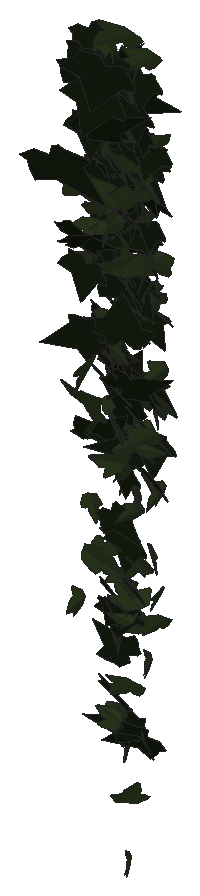
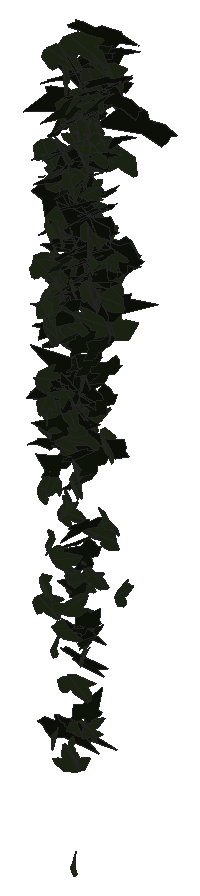
# SketchUp Ruby script. Lengths in millimetres.
U = 1.mm
M = Sketchup.active_model
def pt(a) = Geom::Point3d.new(a.map { |v| v * U })
def face(e, loops, mat)
  f = e.add_face(loops[0].map { |a| pt(a) })
  loops[1..].each { |l| e.add_face(l.map { |a| pt(a) }).erase! }
  f.material = f.back_material = mat if mat
  f
end
# faces: each face lists its corners as indices into pts; further lists are holes
def faces(e, pts, list, mat = nil) = list.each { |f| face(e, (f[0].is_a?(Array) ? f : [f]).map { |l| l.map { |i| pts[i] } }, mat) }
# xy, xz, yz: faces in a plane at the given z, y or x. An outline is a flat list of corners, or four numbers for a rectangle; further outlines are holes
def ring(l) = l.size == 4 ? [[l[0], l[1]], [l[2], l[1]], [l[2], l[3]], [l[0], l[3]]] : l.each_slice(2).to_a
def flat(e, list, mat, &to3) = list.each { |f| face(e, (f[0].is_a?(Array) ? f : [f]).map { |l| ring(l).map { |u, v| to3.(u, v) } }, mat) }
def xy(e, z, list, mat = nil) = flat(e, list, mat) { |x, y| [x, y, z] }
def xz(e, y, list, mat = nil) = flat(e, list, mat) { |x, z| [x, y, z] }
def yz(e, x, list, mat = nil) = flat(e, list, mat) { |y, z| [x, y, z] }
def lines(e, pts, list) = list.each { |a, b| e.add_line(pt(pts[a]), pt(pts[b])) }
# prism: a flat outline (further loops are holes) pulled along v
def prism(e, loops, v, mat = nil)
  f = face(e, loops, mat); d = Geom::Vector3d.new(v.map { |x| x * U })
  f.pushpull(f.normal.samedirection?(d) ? d.length : -d.length)
end
def box(e, o, s, mat = nil) = prism(e, [[o, [o[0] + s[0], o[1], o[2]], [o[0] + s[0], o[1] + s[1], o[2]], [o[0], o[1] + s[1], o[2]]]], [0, 0, s[2]], mat)
def at(x, y, z, deg = 0) = Geom::Transformation.translation(pt([x, y, z])) * Geom::Transformation.rotation(ORIGIN, Z_AXIS, deg.degrees)
def axes(o, x, y, z) = Geom::Transformation.new([*x, 0, *y, 0, *z, 0, *pt(o).to_a, 1])
def part(name) = M.definitions.add(name)
# library, detail: a bought-in or finely detailed component or shape, given as its bounding box
def library(name, o, s) = part(name).tap { |d| box(d.entities, o, s) }
def detail(e, o, s) = box(e.add_group.entities, o, s)
def put(e, d, t, mat = nil) = e.add_instance(d, t).tap { |i| i.material = mat if mat }
def group(e, t, mat = nil) = e.add_group.tap { |g| g.transformation = t; g.material = mat if mat }.entities
root = M.entities
M.materials.add("efeu1").color = [18, 25, 13]
M.materials.add("efeu2").color = [43, 57, 29]
c1 = part("ivyleaf_9")
p = [[39.1,54.8,31.7],[34.5,51.8,30.2],[-5.3,25.2,17.3],[-17.9,28.3,20.9],[-21.6,21.7,17],[-20.2,4.3,5.3],
  [-22.9,-0.3,2.5],[-17.1,-4,-0.6],[-2,-2.1,-1.2],[-0.7,-15.4,-10.1],[16.6,-22.3,-16.7],[21.1,-15.1,-12.5],
  [32.7,-10.7,-11],[46.1,-1.8,-6.6],[30.8,11.2,3.8]]
faces(c1.entities,p,[[0,1,2,3,4,5,6,7,8,9,10,11,12,13,14]],"efeu1")
c2 = part("ivyleaf_10")
p = [[0,12.8,-0.8],[-1.5,51.3,-10.9],[-4.9,51,-11.6],[-13.6,26.5,-7.3],[-13.2,15.9,-4.6],[-21.1,19.3,-7.2],
  [-29.5,16.3,-8.3],[-29.2,8.3,-6.2],[-19.7,-9.8,0.5],[-7.6,-13,4],[1,-12.2,5.8],[-0.4,51.1,-11.1],
  [-1.5,51.1,-10.9],[1,-12.4,5.9],[16.9,-12.4,3.5],[35.1,9.1,-5.1],[35,12.9,-6.1],[20.5,16.4,-4.9],
  [15.8,15,-3.8],[15.3,27.6,-7.1],[12.8,31.3,-7.8]]
faces(c2.entities,p,[[0,1,2,3,4,5,6,7,8,9,10],[11,12,0,13,14,15,16,17,18,19,20]],"efeu2")
put(root,c1,axes([1689.7,958.4,1591.8],[0.18175,-0.69118,-0.44409],[0.28373,0.45424,-0.67492],[1.53762,-0.00212,0.17703]))
put(root,c2,axes([1712.9,944.8,861.4],[0.26339,-0.83853,-0.06256],[-0.02165,0.06153,-0.84988],[1.60018,0.13885,-0.0012]))
put(root,c2,axes([1714.8,968.7,1227.5],[-0.08093,-0.75345,0.21901],[-0.01981,-0.21877,-0.75464],[1.49318,-0.04374,0.00186]))
put(root,c1,axes([1697.6,934.2,1567.8],[0.12261,-0.83473,-0.10782],[-0.03969,0.10651,-0.83712],[1.60137,0.06655,-0.01249]))
put(root,c2,axes([1698,951.7,701.3],[0.88646,-0.26689,0.42385],[0.67692,-0.2313,-0.53649],[0.67121,0.58574,-0.01872]))
put(root,c2,axes([1707.4,908.3,531.4],[-0.11115,-0.03435,0.82545],[0.45417,-0.79293,-0.01611],[1.50533,0.2367,0.06581]))
put(root,c2,axes([1718.6,970.6,1290.3],[-0.64483,-0.74743,0.17146],[-0.05891,-0.17397,-0.81952],[1.45826,-0.33753,0.04271]))
put(root,c2,axes([1712.3,947.3,1230.7],[1.40107,0.27254,-0.1564],[-0.2771,-0.0572,-0.78499],[-0.52997,0.75042,-0.00303]))
put(root,c2,axes([1681.9,953.9,1146.6],[0.09509,-0.01483,0.82486],[1.55484,0.11589,-0.0474],[-0.21851,0.8182,0.02167]))
put(root,c1,axes([1683.9,924.1,1209.7],[0.19618,-0.20205,0.79884],[1.13632,-0.53653,-0.21274],[1.0808,0.60076,0.07867]))
put(root,c2,axes([1694.1,979.8,590.5],[0.81213,-0.23414,-0.46095],[0.7643,-0.22632,0.48672],[-0.61972,-0.58596,-0.0038]))
put(root,c2,axes([1720.6,981.4,1172.7],[-0.21338,-0.76033,0.12533],[-0.03901,-0.12367,-0.76855],[1.46607,-0.11395,-0.00221]))
put(root,c1,axes([1730.8,969.3,1173.4],[-1.32931,-0.39113,0.2691],[0.46256,0.11663,0.80036],[-0.77619,0.73936,0.0161]))
put(root,c1,axes([1692.7,909.5,1210.1],[0.96541,0.73315,-0.17413],[0.18159,0.14573,0.89151],[1.4226,-0.51613,0.00437]))
put(root,c1,axes([1694.9,924,1540.4],[-0.51678,-0.22066,-0.81665],[1.50326,0.24095,-0.32773],[0.57643,-0.82619,0.12253]))
put(root,c1,axes([1697.5,958.3,998.7],[0.37662,-0.72797,0.42536],[0.33819,-0.3911,-0.752],[1.56862,0.2591,0.06]))
put(root,c2,axes([1716.9,959.8,1362.8],[0.0056,0.02601,-0.84155],[0.42991,0.81068,0.02585],[1.54365,-0.22587,-0.00415]))
put(root,c1,axes([1694.8,968.2,942.3],[0.78274,-0.63319,0.40762],[0.43873,-0.33629,-0.75498],[1.3644,0.47139,0.00892]))
put(root,c2,axes([1725.9,907.7,1570.8],[0.01398,-0.83915,0.07771],[0.00221,-0.07771,-0.83918],[1.6039,0.00742,0.00048]))
put(root,c1,axes([1706.2,972.5,1047.1],[0.19524,-0.63407,0.45046],[0.11585,-0.44642,-0.64225],[1.47575,0.11893,-0.00918]))
put(root,c1,axes([1709.6,989,479.4],[0.66706,-0.35539,-0.59071],[0.74817,-0.44134,0.49877],[-1.07779,-0.52632,-0.01937]))
put(root,c2,axes([1725,969.4,1276.2],[0.09274,-0.68093,-0.48319],[0.05434,0.48508,-0.68073],[1.58814,0.02316,0.05151]))
put(root,c2,axes([1725.1,975.1,1174.3],[0.89988,-0.63868,-0.11348],[-0.09706,0.10339,-0.79439],[1.23074,0.47513,0.02032]))
put(root,c1,axes([1716.6,914.3,1171.3],[-0.44413,-0.81643,0.19969],[-0.07124,-0.19695,-0.84894],[1.59805,-0.23568,0.01765]))
put(root,c1,axes([1721.5,989.8,319.3],[0.82818,-0.67144,-0.05441],[0.06196,-0.04374,0.80011],[-1.28057,-0.43636,0.00352]))
put(root,c1,axes([1716.6,976.2,1198.5],[-0.32791,-0.69422,0.4045],[-0.00427,-0.41328,-0.71024],[1.52916,-0.15002,0.08476]))
put(root,c1,axes([1714.3,982.9,1320.9],[-0.00979,-0.79459,-0.01398],[-0.00021,0.01399,-0.79461],[1.5125,-0.00514,-0.0002]))
put(root,c1,axes([1703,980.8,825.3],[0.57062,-0.68673,0.3923],[0.36422,-0.34408,-0.74858],[1.46048,0.35412,0.03341]))
put(root,c1,axes([1721,921.5,1440.8],[-0.45029,-0.78834,0.02024],[-0.00973,-0.0196,-0.82308],[1.50083,-0.23665,0.00074]))
put(root,c2,axes([1723.1,950.8,1264.9],[-0.90653,-0.68564,0.09174],[0.13397,0.06276,0.83457],[-1.30971,0.48099,0.02187]))
put(root,c1,axes([1718.5,995.4,1203.8],[-0.17542,-0.66346,0.40385],[-0.03397,-0.40476,-0.66905],[1.47784,-0.08806,0.03256]))
put(root,c1,axes([1726.3,961.8,1426.7],[-0.70275,-0.70041,0.04303],[-0.02428,-0.04191,-0.79174],[1.33532,-0.36938,0.00825]))
put(root,c1,axes([1714.1,958,1322.9],[0.20442,-0.71739,-0.34234],[0.01173,0.34619,-0.72352],[1.51277,0.09426,0.05187]))
put(root,c1,axes([1714.5,979.5,1246.9],[-0.05502,-0.70997,-0.30148],[0.22795,0.2939,-0.70361],[1.45019,-0.07313,0.09916]))
put(root,c1,axes([1711.7,994.8,505.4],[0.0111,-0.47755,0.6402],[0.33689,-0.62352,-0.46672],[1.48227,0.14529,0.10128]))
put(root,c1,axes([1756.8,971.7,418],[-1.3002,0.00659,-0.40656],[-0.77375,0.0026,0.6832],[0.0133,0.79498,0.00113]))
put(root,c2,axes([1734.7,969.3,1202.3],[0.53911,-0.66026,-0.3094],[-0.12299,0.30789,-0.7162],[1.38227,0.28491,0.05695]))
put(root,c1,axes([1719.2,968.4,1183.5],[1.46545,0.1758,0.2885],[-0.53773,-0.05857,0.78979],[0.35252,-0.82017,0.00544]))
put(root,c1,axes([1703.3,963.2,1259.9],[1.4237,-0.12324,0.3191],[0.59676,-0.05966,-0.7581],[0.26023,0.81108,-0.00728]))
put(root,c1,axes([1716.2,943,829.9],[-0.70545,-0.1078,0.73364],[1.40662,-0.12015,0.35576],[0.11433,0.81313,0.14983]))
put(root,c1,axes([1719.5,949.1,1340],[-0.06274,-0.76151,0.28992],[0.10539,-0.29158,-0.75957],[1.5472,-0.01102,0.0635]))
put(root,c1,axes([1715.1,982.5,1019],[0.28871,-0.66109,0.46611],[0.15423,-0.45943,-0.67798],[1.53173,0.17087,-0.01959]))
put(root,c2,axes([1742.7,975.7,277.2],[0.56167,0.54373,0.45632],[-0.41077,-0.40205,0.61866],[1.28701,-0.36562,-0.00169]))
put(root,c2,axes([1722.2,986.1,294.7],[0.97846,-0.29877,0.32403],[0.53817,-0.15829,-0.5946],[0.64344,0.58673,0.00459]))
put(root,c1,axes([1721.8,958.5,1509.5],[0.02552,-0.80973,0.16957],[0.01297,-0.16948,-0.80983],[1.57445,0.01452,0.00392]))
put(root,c1,axes([1725.2,968.3,1283.7],[-0.91337,0.32252,0.60719],[0.78652,-0.45647,0.56909],[1.04576,0.62501,0.10231]))
put(root,c1,axes([1717.4,970.4,1280.6],[-0.56151,-0.10121,0.8328],[1.58885,0.05168,0.30204],[-0.15752,0.882,0.07787]))
put(root,c2,axes([1728.5,987.5,431.1],[-0.39373,0.19724,0.66334],[0.60116,-0.58911,0.27368],[1.1719,0.36846,0.08247]))
put(root,c2,axes([1728.5,958.7,1446],[0.25264,0.27585,-0.84181],[0.57161,0.78678,0.30518],[1.5861,-0.32748,0.02411]))
put(root,c2,axes([1754.6,968.9,568.4],[-0.60968,-0.19606,-0.6035],[-0.97342,-0.32036,0.37557],[-0.71481,0.60349,0.0033]))
put(root,c1,axes([1769.6,972.8,276.3],[-0.91405,0.24968,0.55378],[-0.93529,0.25528,-0.5413],[-0.67961,-0.68714,0.00012]))
put(root,c2,axes([1741.4,976.4,1441.1],[0.40827,-0.78435,0.05426],[0.0332,-0.05148,-0.81315],[1.49598,0.2152,0.00324]))
put(root,c1,axes([1733.9,996.6,1221.4],[-0.46341,-0.77579,0.29791],[-0.07884,-0.29871,-0.81175],[1.57964,-0.2425,0.04688]))
put(root,c1,axes([1740.8,988.5,490.6],[-1.25205,-0.20013,-0.33798],[0.61416,0.10049,-0.68763],[0.42619,-0.73275,-0.002]))
put(root,c2,axes([1743.6,964.1,1490.1],[0.45172,-0.77855,-0.13077],[-0.05376,0.12809,-0.81386],[1.50153,0.2388,0.0102]))
put(root,c1,axes([1737.9,994.4,1338.5],[-0.62766,-0.68595,0.20589],[-0.07877,-0.20803,-0.7594],[1.36076,-0.32844,0.05101]))
put(root,c1,axes([1727.9,974.1,1162.2],[-0.2298,-0.75737,-0.28282],[0.19594,0.26923,-0.76491],[1.52612,-0.14861,0.05562]))
put(root,c2,axes([1744.7,939.4,1303.3],[0.00013,-0.7838,0.19781],[0.03443,-0.19776,-0.78361],[1.53812,0.00449,0.01752]))
put(root,c2,axes([1746.2,960.2,996.6],[0.46696,-0.40291,-0.73346],[-0.09245,0.75618,-0.43165],[1.58998,0.1623,0.19031]))
put(root,c2,axes([1732.1,937.6,1470.7],[0.68586,-0.63469,0.58028],[0.65757,-0.4693,-0.72788],[1.4988,0.49634,0.0538]))
put(root,c2,axes([1745.3,955.2,980.4],[0.39551,-0.69335,0.09716],[0.06013,-0.09196,-0.72381],[1.33111,0.21017,0.00383]))
put(root,c2,axes([1722,985.9,880.1],[1.06849,-0.05936,0.54914],[1.04372,-0.0334,-0.56427],[0.12526,0.78462,0.01753]))
put(root,c1,axes([1724.3,952.9,1526.3],[0.79877,-0.79627,0.01693],[0.0145,-0.01512,-0.9001],[1.51573,0.41977,-0.00031]))
put(root,c1,axes([1755.9,987.7,944.3],[-1.19985,0.38707,-0.37531],[0.60775,-0.19719,-0.73978],[-0.82676,-0.7067,0.00086]))
put(root,c1,axes([1738.6,944.7,1310.7],[-0.15614,0.39346,0.74912],[-0.18365,-0.75207,0.38445],[1.59991,-0.04793,0.11724]))
put(root,c1,axes([1757.8,874.5,1074.2],[-0.07594,-0.47857,-0.87325],[0.19127,-0.87143,0.47297],[-1.88551,-0.06912,0.08315]))
put(root,c1,axes([1759.8,973.4,820.1],[-0.11583,-0.62189,-0.43502],[-0.09973,-0.43193,0.62481],[-1.44097,0.07989,-0.00827]))
put(root,c2,axes([1736.4,955.2,1301.4],[-0.2989,0.26463,0.78438],[0.77093,-0.6717,0.30772],[1.374,0.43445,-0.00202]))
put(root,c2,axes([1757.2,974.1,1286.5],[-0.60406,-0.62272,0.34803],[-0.21433,-0.33241,-0.69747],[1.34067,-0.33372,0.04531]))
put(root,c1,axes([1724,985.9,1065.8],[0.83335,-0.63856,0.29211],[0.30085,-0.24577,-0.77422],[1.30212,0.46546,-0.00807]))
put(root,c2,axes([1721.9,963.2,1436.4],[1.15835,-0.03301,0.65341],[1.24352,-0.01495,-0.60937],[0.06365,0.89283,0.01395]))
put(root,c1,axes([1746.9,970.3,1545.8],[-0.63528,-0.74643,0.16803],[-0.00823,-0.18148,-0.81477],[1.45612,-0.32668,0.0687]))
put(root,c2,axes([1743.4,951.7,1537.2],[-0.70265,-0.4983,-0.65806],[0.67983,0.55344,-0.61948],[1.41626,-0.51288,-0.02912]))
put(root,c1,axes([1738.5,957.3,687.7],[0.32761,-0.5842,-0.53926],[-0.15922,0.53539,-0.60671],[1.50473,0.18384,0.05321]))
put(root,c1,axes([1735.1,941.7,1527.1],[0.31322,-0.75663,-0.3218],[0.05471,0.33328,-0.76891],[1.56389,0.13988,0.09135]))
put(root,c2,axes([1768.2,967.2,364.2],[-0.95032,-0.27935,0.38802],[-0.63465,-0.1986,-0.57209],[0.6521,-0.60037,0.0087]))
put(root,c2,axes([1756.5,963.3,1482.4],[0.88185,-0.51135,-0.45805],[-0.17449,0.50157,-0.65269],[1.29485,0.41584,0.224]))
put(root,c1,axes([1727.7,968.1,626.1],[0.80692,-0.59008,0.34279],[0.35305,-0.28871,-0.72643],[1.24988,0.46251,-0.01611]))
put(root,c2,axes([1745,994.8,243],[0.59429,-0.53217,0.51218],[0.49076,-0.44253,-0.61701],[1.31725,0.40496,-0.0012]))
put(root,c2,axes([1757.1,926,1558.8],[-0.47647,-0.89449,-0.17919],[0.08701,0.17328,-0.92886],[1.73404,-0.25448,-0.00263]))
put(root,c1,axes([1776.6,961.1,884.9],[-0.04519,0.05329,0.85173],[-0.77536,0.74799,-0.05816],[-1.42715,-0.40807,0.00462]))
put(root,c2,axes([1757.9,968.2,1205.8],[-0.26066,0.64036,0.37512],[-0.39872,0.33258,-0.64423],[-1.355,-0.22105,0.11741]))
put(root,c1,axes([1722.6,968,966.7],[1.30364,-0.22833,0.42596],[0.78395,-0.11064,-0.7217],[0.48111,0.79899,0.02179]))
put(root,c1,axes([1747,980.5,1501],[-0.22377,-0.802,0.12552],[-0.04862,-0.12311,-0.81054],[1.54418,-0.12009,-0.00733]))
put(root,c1,axes([1734.4,973.8,571.3],[0.65266,-0.66391,0.2397],[0.24123,-0.20423,-0.74702],[1.32154,0.36516,0.01799]))
put(root,c2,axes([1763.9,983.8,513.7],[0.72844,0.68648,0.29535],[-0.30241,-0.24949,0.7858],[1.38977,-0.4141,0.01618]))
put(root,c2,axes([1773.1,984.8,469.9],[0.40202,0.25243,0.6061],[-0.75972,-0.45613,0.32909],[0.99211,-0.45158,0.0064]))
put(root,c2,axes([1754.6,938.9,1255.9],[0.15552,-0.302,-0.79484],[0.33589,0.78714,-0.28093],[1.58301,-0.13735,0.1377]))
put(root,c1,axes([1734.8,914.6,1067.5],[0.16697,-0.14272,-0.8229],[1.49898,-0.26113,0.12926],[-0.5288,-0.78528,0.10657]))
put(root,c2,axes([1781.8,938.2,1624.7],[-0.93444,-0.35359,0.63048],[-1.00895,-0.34199,-0.60464],[0.93524,-0.72222,-0.02236]))
put(root,c1,axes([1754.8,969.6,940],[-1.03618,0.47702,0.31955],[0.46198,-0.20784,0.72385],[0.99028,0.59609,-0.00333]))
put(root,c2,axes([1747.4,988.9,10.5],[0.05223,-0.07451,0.68136],[0.69502,-0.57547,-0.07764],[1.10392,0.36584,0.01665]))
put(root,c2,axes([1762.8,977.7,1380.4],[-0.27451,-0.79271,-0.04404],[0.01899,0.04295,-0.80573],[1.5109,-0.14456,0.00213]))
put(root,c1,axes([1772.7,934.8,1348.9],[0.88871,0.12425,-0.72216],[-1.35761,-0.11885,-0.4817],[-0.31909,0.85172,0.03813]))
put(root,c2,axes([1776.8,976.5,917.6],[-1.15502,0.13325,0.44916],[-0.83127,0.10498,-0.6213],[-0.32256,-0.74768,-0.00718]))
put(root,c1,axes([1744.6,963.5,1006.2],[0.15391,-0.70528,0.31233],[0.14915,-0.3049,-0.7088],[1.46042,0.10547,0.03947]))
put(root,c2,axes([1763.9,979.3,1303.3],[-1.34956,-0.36715,-0.06502],[0.10981,0.02998,-0.79851],[0.70108,-0.71145,-0.00009]))
put(root,c1,axes([1750.2,971.7,768],[-0.17442,-0.66778,0.37274],[0.08356,-0.37939,-0.66888],[1.4531,-0.05834,0.0832]))
put(root,c1,axes([1728.5,807.1,1429.7],[-0.28314,-0.30864,-1.04293],[1.57429,0.65139,-0.31076],[1.34408,-0.82797,0.14429]))
put(root,c2,axes([1750.6,981.5,945.8],[1.10286,0.51038,0.1776],[0.24058,0.12515,-0.77213],[-0.99995,0.59302,0.0101]))
put(root,c2,axes([1759.2,971.9,766],[0.3613,-0.66091,0.34813],[0.27021,-0.32073,-0.68631],[1.39577,0.23317,0.04275]))
put(root,c2,axes([1772.4,934.1,1469.3],[-1.58699,0.14332,0.18917],[-0.35391,0.03485,-0.84607],[-0.28066,-0.85433,-0.00278]))
put(root,c2,axes([1746.6,930.1,1601.3],[1.03095,-0.4128,0.53936],[0.8131,-0.32923,-0.68106],[1.00491,0.68989,-0.00228]))
put(root,c2,axes([1751.8,971.3,547.7],[-0.91798,0.13534,0.4645],[0.82941,-0.16334,0.50012],[0.39992,0.64941,0.02899]))
put(root,c2,axes([1754.8,937.9,1429.4],[-1.3764,-0.33241,0.3256],[0.58506,0.11041,0.79552],[-0.66479,0.7854,0.02598]))
put(root,c1,axes([1760.5,951.8,1364.9],[-0.55817,-0.68596,0.31961],[-0.00659,-0.34156,-0.73623],[1.44026,-0.2674,0.1205]))
put(root,c1,axes([1752.6,979.7,1493.2],[0.05627,-0.82043,0.0385],[-0.00986,-0.03871,-0.82094],[1.56313,0.02929,-0.00656]))
put(root,c1,axes([1742.2,985.5,963.7],[0.43339,-0.13195,-0.80412],[1.39862,-0.32752,0.26185],[-0.67013,-0.76889,0.02646]))
put(root,c2,axes([1771.9,944.2,1212.1],[0.80261,-0.55874,-0.39346],[-0.24454,0.38927,-0.69051],[1.2774,0.42558,0.11503]))
put(root,c1,axes([1746.3,953.4,1322],[1.49653,-0.27011,-0.05779],[-0.09921,0.02613,-0.83139],[0.51627,0.78801,0.00775]))
put(root,c1,axes([1737.2,931.2,1035.1],[0.42058,-0.49408,0.66016],[0.86878,-0.49587,-0.52393],[1.30693,0.48863,0.13583]))
put(root,c1,axes([1747.7,953.2,1415.4],[-0.35849,-0.53119,-0.68217],[0.78234,0.5592,-0.54893],[1.44761,-0.43375,0.12773]))
put(root,c1,axes([1755.5,986.3,1361.2],[0.1208,-0.75436,0.21104],[-0.00041,-0.21174,-0.75682],[1.49081,0.06106,-0.01731]))
put(root,c2,axes([1737.5,900.4,630.6],[0.28789,-0.04534,0.82537],[1.57078,-0.03832,-0.15336],[0.08738,0.83824,0.03764]))
put(root,c2,axes([1779.2,984.2,1065.2],[-0.68422,-0.60606,0.39445],[-0.27392,-0.37173,-0.70232],[1.34871,-0.38296,0.05747]))
put(root,c2,axes([1743.3,984.2,1096.9],[0.82879,-0.05792,0.65914],[1.23645,-0.11225,-0.43908],[0.23887,0.78199,-0.01421]))
put(root,c2,axes([1790.6,977.3,845.7],[0.48397,0.19286,0.61867],[-1.15278,-0.16551,0.30056],[0.43841,-0.64809,0.10735]))
put(root,c2,axes([1740.7,928.1,1070.4],[-0.31058,0.02788,-0.82667],[1.45202,-0.32042,-0.16141],[-0.60811,-0.77933,0.03679]))
put(root,c1,axes([1774.1,916.1,1467.4],[0.76819,-0.90769,0.0306],[-0.02329,0.02805,0.99339],[-1.72834,-0.40382,0.00021]))
put(root,c2,axes([1761.3,972.6,1165.1],[0.37036,-0.52235,0.60317],[0.64002,-0.50932,-0.54957],[1.37713,0.37719,0.0932]))
put(root,c1,axes([1754.2,976.7,1522.2],[1.14301,-0.47896,-0.30462],[-0.27086,0.30225,-0.75583],[1.04579,0.60177,0.13718]))
put(root,c2,axes([1760.7,985,731.5],[-0.19833,0.29403,-0.60238],[0.38186,-0.56798,-0.31195],[-1.21723,-0.22609,0.00029]))
put(root,c2,axes([1776.5,944.5,794.8],[0.14461,-0.79622,-0.29415],[-0.06073,0.29244,-0.79983],[1.61433,0.08233,-0.00374]))
put(root,c1,axes([1794.6,954.9,830.5],[-0.24483,-0.31702,-0.71842],[-0.60133,-0.64557,0.34145],[-1.36819,0.34046,-0.02151]))
put(root,c2,axes([1779.4,971.3,699.3],[-0.09188,-0.35832,0.57818],[-0.1832,-0.5702,-0.36142],[1.28154,-0.1072,-0.01021]))
put(root,c1,axes([1765.9,964.1,640.7],[-0.34445,-0.75598,0.18495],[-0.04995,-0.18385,-0.77716],[1.48037,-0.18211,0.01681]))
put(root,c1,axes([1761.5,984.8,1231.1],[0.00631,-0.75327,-0.10452],[0.01031,0.10454,-0.75325],[1.44732,0.00254,0.00582]))
put(root,c2,axes([1781.8,968.8,716.7],[-0.1642,0.16478,0.66581],[-0.62027,0.58061,-0.18592],[-1.14861,-0.3371,0.00522]))
put(root,c2,axes([1783,951.9,1507.6],[-0.90212,-0.58104,0.39007],[-0.17718,-0.41458,-0.73069],[1.32008,-0.45272,0.16849]))
put(root,c1,axes([1798.7,970,272.3],[0.08273,0.05773,-0.77306],[-1.16622,-0.4717,-0.06968],[-0.9037,0.61401,0.01915]))
put(root,c1,axes([1755.5,902.3,1587.1],[0.88544,-0.7141,-0.10338],[-0.08976,0.09265,-0.85221],[1.37031,0.46749,0.01098]))
put(root,c1,axes([1778.7,933.3,1360.5],[0.50933,0.81005,0.16758],[0.11839,0.15592,-0.85305],[-1.56987,0.27457,-0.00996]))
put(root,c2,axes([1777.5,922.8,1393.4],[-1.59029,0.17919,-0.02298],[0.04268,-0.00499,-0.85458],[-0.34116,-0.83589,0.00018]))
put(root,c2,axes([1798.1,967.4,597.8],[-0.77282,0.21039,-0.52397],[-0.95134,0.1662,0.45411],[0.49976,0.64173,0.05418]))
put(root,c1,axes([1767.2,940.9,1555.6],[-0.23873,0.72562,0.44241],[0.05128,-0.44359,0.73518],[1.61663,0.12122,0.04201]))
put(root,c2,axes([1763.5,851,1369],[-1.43791,-0.27252,-0.60479],[1.06574,0.22939,-0.80291],[0.67682,-0.94019,-0.0206]))
put(root,c1,axes([1773.1,976.1,1281.2],[-0.80432,0.20859,-0.65759],[1.16152,-0.24653,-0.47042],[-0.6122,-0.74179,-0.02858]))
put(root,c1,axes([1765.7,976,1136],[0.12419,-0.7069,0.31374],[0.00211,-0.31477,-0.70945],[1.47193,0.0601,-0.02546]))
put(root,c1,axes([1799.2,974.3,1230.3],[-1.19845,-0.27747,0.39813],[-0.70033,-0.15219,-0.68808],[0.6021,-0.72929,-0.00788]))
put(root,c1,axes([1766.2,984.4,1377],[0.11253,-0.80207,0.0263],[0.00457,-0.0262,-0.80425],[1.52731,0.05917,0.00047]))
put(root,c1,axes([1765,945.9,1392.1],[0.54003,-0.47267,-0.59942],[-0.15569,0.61698,-0.52524],[1.44446,0.24321,0.16749]))
put(root,c1,axes([1766.3,905.2,1585.3],[0.02859,-0.75793,-0.37824],[0.07797,0.3785,-0.75684],[1.61026,-0.00487,0.04336]))
put(root,c2,axes([1790.7,935.8,1329.3],[-1.33896,-0.48754,0.09608],[-0.14943,-0.05538,-0.85595],[0.93386,-0.7079,0.00079]))
put(root,c1,axes([1767.7,976.1,1158],[0.68393,-0.59923,-0.3386],[-0.20326,0.3288,-0.69523],[1.29406,0.36835,0.06975]))
put(root,c2,axes([1789,969.9,1122.7],[-0.42541,-0.72706,0.15668],[-0.04907,-0.15593,-0.76036],[1.41466,-0.22405,0.02074]))
put(root,c2,axes([1762.9,917,1038.3],[-0.38393,0.08556,-0.81779],[0.93918,-0.66094,-0.19087],[-1.25175,-0.52214,0.10761]))
put(root,c1,axes([1774.4,992.2,1051.6],[-0.31208,-0.64872,0.4484],[0.19907,-0.47184,-0.64438],[1.48762,-0.07295,0.1803]))
put(root,c2,axes([1791.1,956.3,834],[0.01018,0.07548,0.79166],[-0.03909,-0.7914,0.07559],[1.51301,-0.02096,-0.00338]))
put(root,c2,axes([1786.7,900.9,903.5],[-0.91318,0.69752,0.08512],[-0.09427,0.06925,-0.84661],[-1.33404,-0.48236,0.00156]))
put(root,c1,axes([1768.4,948.9,1144.4],[-0.46496,-0.53499,-0.67189],[0.77265,0.54365,-0.58049],[1.44045,-0.46429,0.09449]))
put(root,c2,axes([1790.3,957.1,1568.5],[0.49057,-0.65205,-0.46729],[-0.03224,0.48629,-0.6879],[1.52641,0.21983,0.13566]))
put(root,c1,axes([1802.7,957.7,1324.7],[0.69233,0.00093,-0.774],[-1.47068,0.04919,-0.36312],[0.08397,0.85381,0.02176]))
put(root,c2,axes([1793.2,959.1,1270.9],[-0.02216,-0.75078,-0.43594],[0.02052,0.43582,-0.75087],[1.65217,-0.01548,0.00348]))
put(root,c1,axes([1761.1,981.2,1111],[0.98909,-0.53509,0.37932],[0.47405,-0.2867,-0.7457],[1.15481,0.576,-0.01878]))
put(root,c2,axes([1794.7,986.8,1088.2],[-0.40688,-0.70046,0.08652],[-0.02589,-0.0863,-0.73226],[1.34299,-0.21388,0.01209]))
put(root,c1,axes([1773.3,987.1,1205],[0.31708,-0.75373,0.15222],[0.07874,-0.14674,-0.77188],[1.46134,0.17145,0.00856]))
put(root,c2,axes([1790.9,968.6,1422.5],[0.89049,-0.68621,-0.01716],[-0.01336,0.01598,-0.83054],[1.30634,0.46793,0.00321]))
put(root,c1,axes([1785.9,985.3,1417.9],[-0.42312,-0.62429,0.45999],[-0.06509,-0.47016,-0.65463],[1.47441,-0.19991,0.10311]))
put(root,c2,axes([1807.2,888.6,836.5],[-0.3613,-0.2558,-0.80001],[-0.93381,-0.63191,0.31848],[-1.29739,0.52606,-0.00644]))
put(root,c2,axes([1783.5,886,1439.8],[0.45018,-0.91313,-0.24005],[0.11177,-0.23276,0.94327],[-1.79343,-0.24372,-0.00147]))
put(root,c2,axes([1800.5,968.9,264.4],[-0.67794,0.53889,0.4395],[-0.46038,0.36694,-0.64598],[-1.24081,-0.43058,-0.00045]))
put(root,c2,axes([1790,977.9,1155.9],[0.5949,-0.64138,0.30965],[0.29257,-0.26944,-0.71326],[1.32355,0.34784,0.01849]))
put(root,c2,axes([1802.1,985.3,1111],[-0.78076,-0.69039,0.14792],[-0.12103,-0.13425,-0.80296],[1.33832,-0.41491,0.01368]))
put(root,c2,axes([1797.3,991.1,1085.6],[-0.11909,-0.70016,0.30085],[0.12632,-0.30572,-0.69769],[1.44484,-0.03098,0.08579]))
put(root,c1,axes([1770.6,981.4,943],[0.14251,-0.04378,-0.84611],[1.57836,-0.16998,0.08219],[-0.32987,-0.83223,0.02772]))
put(root,c2,axes([1793.4,930.7,170.4],[-0.72356,-0.60564,0.09897],[0.106,0.08189,0.71507],[-1.16312,0.38422,0.0036]))
put(root,c1,axes([1789.5,989.5,1372.7],[-0.31732,-0.76447,-0.01786],[0.00526,0.01767,-0.78244],[1.45532,-0.16675,-0.00106]))
put(root,c2,axes([1796.6,980.5,760.6],[-0.96236,0.46782,-0.06119],[0.07643,-0.04669,-0.68883],[-0.89467,-0.5072,0.00697]))
put(root,c1,axes([1799.4,976.1,1372],[-0.76335,-0.58474,0.38684],[-0.11097,-0.4163,-0.68974],[1.32975,-0.37042,0.16451]))
put(root,c1,axes([1800,846.8,1555.3],[-0.99432,-0.87618,0.11869],[-0.12105,-0.10026,-1.02012],[1.67843,-0.5263,-0.00326]))
put(root,c1,axes([1787.5,978.3,1074.7],[-0.27945,-0.59699,-0.45984],[0.31508,0.43149,-0.61304],[1.39913,-0.21641,0.04621]))
put(root,c1,axes([1805.7,900.2,1069.4],[-1.5499,-0.19451,0.51813],[0.95751,0.12392,0.83727],[-0.4389,0.95723,-0.00311]))
put(root,c1,axes([1775.5,976.5,874],[0.87982,-0.63508,0.26605],[0.30004,-0.21431,-0.78551],[1.27564,0.48843,0.00126]))
put(root,c2,axes([1805.9,973.7,1355.8],[-0.27525,-0.10083,0.78985],[0.01181,-0.80289,-0.10135],[1.51539,-0.01206,0.14425]))
put(root,c2,axes([1805.3,989,1123.5],[0.01175,-0.56856,0.52102],[0.01278,-0.52098,-0.5686],[1.46766,0.00909,0.00078]))
put(root,c2,axes([1787.9,936.2,1338.3],[-1.13804,0.25103,0.56603],[0.98099,-0.23423,0.6484],[0.65302,0.78935,0.01239]))
put(root,c2,axes([1818.4,964.6,1187.4],[-1.29094,-0.26558,0.32911],[-0.58836,-0.11308,-0.72841],[0.54921,-0.7454,-0.00676]))
put(root,c2,axes([1771.9,951.1,828.4],[0.29149,-0.01523,-0.79976],[1.51983,-0.04419,0.15377],[-0.08807,-0.81309,0.00662]))
put(root,c2,axes([1805.8,978.1,1271.1],[0.06832,-0.8023,0.25423],[0.08464,-0.2523,-0.80248],[1.59952,0.04762,0.0316]))
put(root,c2,axes([1794,903.7,1192.7],[-0.65877,-0.67975,0.38224],[0.36683,0.33066,0.76256],[-1.43817,0.39571,0.01941]))
put(root,c1,axes([1804.7,853.7,1605.6],[-1.56913,-0.51633,-0.33937],[0.57033,0.16074,-0.97257],[1.02839,-0.87698,0.02155]))
put(root,c1,axes([1783.7,977.1,946.1],[-0.35744,-0.20371,-0.74298],[1.04799,0.49935,-0.2761],[1.02545,-0.58133,0.02319]))
put(root,c2,axes([1822,947.1,1591.7],[-0.61704,-0.47892,0.60739],[-0.53991,-0.53907,-0.57648],[1.36952,-0.4283,0.04639]))
put(root,c2,axes([1796.8,881.7,1297.5],[0.362,-0.33456,0.88892],[0.72704,-0.80307,-0.38399],[1.655,0.42596,-0.02575]))
put(root,c1,axes([1806.3,958.5,1322.7],[1.34734,-0.04043,-0.48017],[-0.91487,0.00016,-0.70873],[0.06385,0.85542,-0.02257]))
put(root,c2,axes([1816.1,990.5,1187.1],[-0.67845,-0.5293,0.39902],[-0.15328,-0.41512,-0.62261],[1.2522,-0.3376,0.13998]))
put(root,c2,axes([1811,995.4,965.7],[-0.08936,-0.26694,0.78899],[0.08399,-0.78992,-0.26463],[1.58299,0.02684,0.05858]))
put(root,c2,axes([1799,979.7,1218.5],[-0.28067,0.33725,-0.66782],[0.30789,-0.65019,-0.36407],[-1.39018,-0.21209,0.0542]))
put(root,c2,axes([1813.4,956.5,1126.5],[0.16689,-0.20611,0.76803],[-0.51438,0.71896,0.2238],[-1.42333,-0.28399,0.00918]))
put(root,c1,axes([1795.4,952.7,1370],[0.45854,-0.76841,-0.33949],[-0.08111,0.34154,-0.80329],[1.59674,0.23801,0.05669]))
put(root,c1,axes([1804.7,979.1,841],[-0.51217,-0.80421,-0.07446],[0.06773,0.0666,-0.84795],[1.53563,-0.27116,0.01257]))
put(root,c1,axes([1787,925.9,954.2],[-0.09958,-0.01524,0.84946],[1.61164,-0.06992,0.0509],[0.13107,0.8482,0.01946]))
put(root,c2,axes([1819.6,979,1420.9],[-0.45864,-0.75874,0.1732],[-0.05091,-0.17314,-0.79565],[1.4803,-0.24103,0.0263]))
put(root,c1,axes([1801.4,951.6,1450.6],[-0.00982,-0.68089,0.51153],[0.00896,-0.51155,-0.68088],[1.6208,-0.0013,0.00686]))
put(root,c2,axes([1805.1,970.9,417.8],[-0.1306,0.04752,0.72748],[0.65568,-0.64185,0.07442],[1.2228,0.34924,0.03779]))
put(root,c1,axes([1784.8,842.6,1484.8],[0.04402,-0.08298,1.0143],[1.90951,0.17177,-0.00883],[-0.32437,0.99992,0.08569]))
put(root,c1,axes([1805.7,971.6,1259.6],[-0.18577,-0.68958,0.36515],[-0.02449,-0.36653,-0.69561],[1.48485,-0.09232,0.03421]))
put(root,c2,axes([1816.8,795.7,1070.7],[0.31562,-1.03656,0.26292],[0.12989,-0.25526,-1.04942],[2.03111,0.1774,0.02625]))
put(root,c2,axes([1800.2,807.7,982.5],[-1.6296,0.15048,0.62072],[1.06977,-0.31547,0.85184],[0.57726,1.00942,0.17368]))
put(root,c1,axes([1808.6,949.4,1550.3],[-0.42385,-0.77074,0.15639],[-0.01216,-0.16076,-0.80138],[1.49672,-0.21957,0.03777]))
put(root,c2,axes([1801.5,992.7,900.4],[0.06588,-0.40899,0.67144],[0.87014,-0.53629,-0.35024],[1.21727,0.40549,0.21402]))
put(root,c1,axes([1794.6,969.5,781.7],[0.40589,-0.59262,0.45455],[0.41761,-0.40214,-0.62724],[1.35872,0.30063,0.057]))
put(root,c1,axes([1813.5,971.2,1403.8],[-0.5714,-0.71781,0.15186],[-0.05935,-0.15145,-0.77753],[1.39512,-0.30044,0.02912]))
put(root,c2,axes([1820,978.4,920.6],[-1.14123,0.36286,0.0569],[-0.10227,0.02109,-0.70081],[-0.69151,-0.60196,0.00974]))
put(root,c2,axes([1810,972.2,632.9],[-0.32088,0.55926,-0.41859],[0.22464,-0.40161,-0.58412],[-1.31039,-0.2058,0.00237]))
put(root,c2,axes([1818.7,983.3,550.8],[0.28537,-0.65208,0.19783],[0.07925,-0.19342,-0.66909],[1.29446,0.15559,-0.00265]))
put(root,c2,axes([1814.3,989.2,741.6],[0.00345,-0.366,0.7582],[0.40428,-0.73347,-0.35457],[1.5505,0.19206,0.09077]))
put(root,c1,axes([1806,936.1,1503.9],[0.14552,0.16267,-0.84513],[-0.11121,0.84749,0.15784],[1.6342,0.04319,0.086]))
put(root,c2,axes([1828.4,972.2,505.5],[-0.49513,-0.54745,0.34009],[-0.27326,-0.30831,-0.60612],[1.19577,-0.29714,0.00231]))
put(root,c2,axes([1832.7,942.6,874.2],[-0.49436,-0.43298,0.49778],[-0.47458,-0.43086,-0.50489],[1.16247,-0.36003,0.00557]))
put(root,c2,axes([1801.6,947.1,1359.8],[-0.65625,0.324,-0.71447],[0.87738,-0.54779,-0.4709],[-1.20807,-0.57384,0.04612]))
put(root,c1,axes([1809.3,923.6,1500.3],[-0.20881,-0.79954,0.25874],[0.09547,-0.2667,-0.80287],[1.59653,-0.08862,0.08185]))
